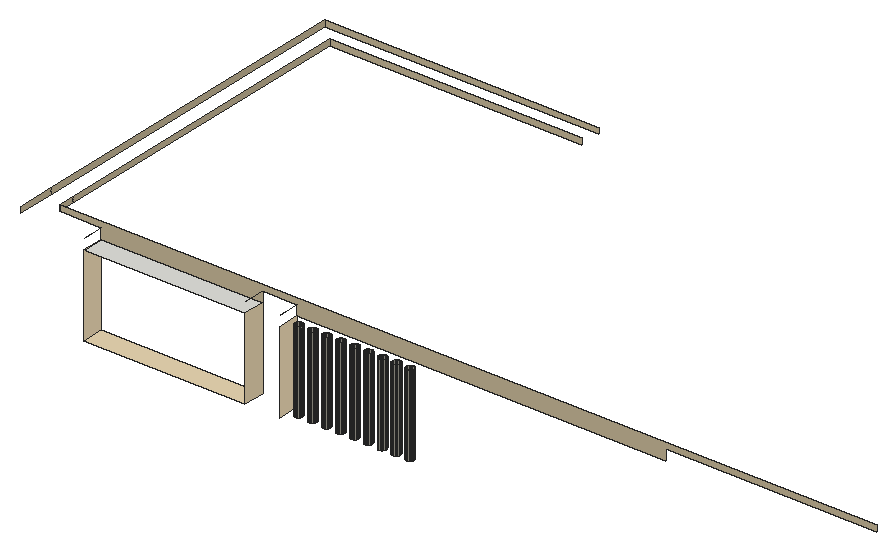
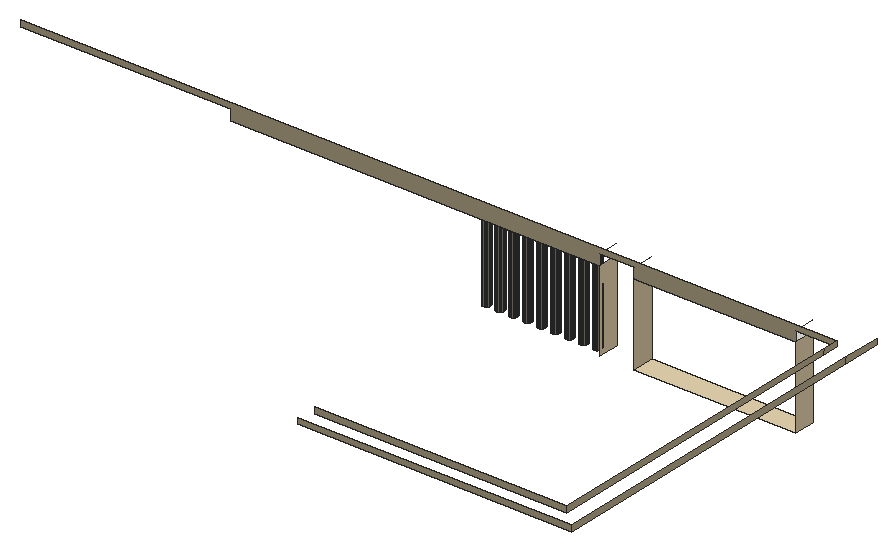
# SketchUp Ruby script. Lengths in inches.
U = 1.inch
M = Sketchup.active_model
def pt(a) = Geom::Point3d.new(a.map { |v| v * U })
def face(e, loops, mat)
  f = e.add_face(loops[0].map { |a| pt(a) })
  loops[1..].each { |l| e.add_face(l.map { |a| pt(a) }).erase! }
  f.material = f.back_material = mat if mat
  f
end
# faces: each face lists its corners as indices into pts; further lists are holes
def faces(e, pts, list, mat = nil) = list.each { |f| face(e, (f[0].is_a?(Array) ? f : [f]).map { |l| l.map { |i| pts[i] } }, mat) }
# xy, xz, yz: faces in a plane at the given z, y or x. An outline is a flat list of corners, or four numbers for a rectangle; further outlines are holes
def ring(l) = l.size == 4 ? [[l[0], l[1]], [l[2], l[1]], [l[2], l[3]], [l[0], l[3]]] : l.each_slice(2).to_a
def flat(e, list, mat, &to3) = list.each { |f| face(e, (f[0].is_a?(Array) ? f : [f]).map { |l| ring(l).map { |u, v| to3.(u, v) } }, mat) }
def xy(e, z, list, mat = nil) = flat(e, list, mat) { |x, y| [x, y, z] }
def xz(e, y, list, mat = nil) = flat(e, list, mat) { |x, z| [x, y, z] }
def yz(e, x, list, mat = nil) = flat(e, list, mat) { |y, z| [x, y, z] }
def lines(e, pts, list) = list.each { |a, b| e.add_line(pt(pts[a]), pt(pts[b])) }
# prism: a flat outline (further loops are holes) pulled along v
def prism(e, loops, v, mat = nil)
  f = face(e, loops, mat); d = Geom::Vector3d.new(v.map { |x| x * U })
  f.pushpull(f.normal.samedirection?(d) ? d.length : -d.length)
end
def box(e, o, s, mat = nil) = prism(e, [[o, [o[0] + s[0], o[1], o[2]], [o[0] + s[0], o[1] + s[1], o[2]], [o[0], o[1] + s[1], o[2]]]], [0, 0, s[2]], mat)
def at(x, y, z, deg = 0) = Geom::Transformation.translation(pt([x, y, z])) * Geom::Transformation.rotation(ORIGIN, Z_AXIS, deg.degrees)
def axes(o, x, y, z) = Geom::Transformation.new([*x, 0, *y, 0, *z, 0, *pt(o).to_a, 1])
def part(name) = M.definitions.add(name)
# library, detail: a bought-in or finely detailed component or shape, given as its bounding box
def library(name, o, s) = part(name).tap { |d| box(d.entities, o, s) }
def detail(e, o, s) = box(e.add_group.entities, o, s)
def put(e, d, t, mat = nil) = e.add_instance(d, t).tap { |i| i.material = mat if mat }
def group(e, t, mat = nil) = e.add_group.tap { |g| g.transformation = t; g.material = mat if mat }.entities
root = M.entities
M.materials.add("[Formica Graystone]").color = [149, 146, 135]
M.materials.add("[Quartz Light Brown]").color = [242, 223, 185]
M.materials.add("[Quartz Light Brown]1").color = [234, 216, 179]
M.materials.add("[Quartz Light Brown]2").color = [199, 184, 152]
xy(root,552.75,[[185.125,21.93,184.41,22.02,183.75,22.3,183.18,22.74,182.74,23.3,182.47,23.97,182.375,24.68,182.47,25.39,182.74,26.05,183.18,26.625,183.75,27.0625,184.41,27.34,185.125,27.43,185.84,27.34,186.5,27.0625,187.07,26.625,187.51,26.05,187.78,25.39,187.875,24.68,187.78,23.97,187.51,23.3,187.07,22.74,186.5,22.3,185.84,22.02],[194.6875,21.93,193.98,22.02,193.3125,22.3,192.74,22.74,192.31,23.3,192.03,23.97,191.9375,24.68,192.03,25.39,192.31,26.05,192.74,26.625,193.3125,27.0625,193.98,27.34,194.6875,27.43,195.4,27.34,196.0625,27.0625,196.63,26.625,197.07,26.05,197.34,25.39,197.4375,24.68,197.34,23.97,197.07,23.3,196.63,22.74,196.0625,22.3,195.4,22.02],[204.25,21.93,203.54,22.02,202.875,22.3,202.31,22.74,201.87,23.3,201.59,23.97,201.5,24.68,201.59,25.39,201.87,26.05,202.31,26.625,202.875,27.0625,203.54,27.34,204.25,27.43,204.96,27.34,205.625,27.0625,206.19,26.625,206.63,26.05,206.91,25.39,207,24.68,206.91,23.97,206.63,23.3,206.19,22.74,205.625,22.3,204.96,22.02],[213.8125,21.93,213.1,22.02,212.4375,22.3,211.87,22.74,211.43,23.3,211.16,23.97,211.0625,24.68,211.16,25.39,211.43,26.05,211.87,26.625,212.4375,27.0625,213.1,27.34,213.8125,27.43,214.52,27.34,215.1875,27.0625,215.76,26.625,216.19,26.05,216.47,25.39,216.5625,24.68,216.47,23.97,216.19,23.3,215.76,22.74,215.1875,22.3,214.52,22.02],[223.375,21.93,222.66,22.02,222,22.3,221.43,22.74,220.99,23.3,220.72,23.97,220.625,24.68,220.72,25.39,220.99,26.05,221.43,26.625,222,27.0625,222.66,27.34,223.375,27.43,224.09,27.34,224.75,27.0625,225.32,26.625,225.76,26.05,226.03,25.39,226.125,24.68,226.03,23.97,225.76,23.3,225.32,22.74,224.75,22.3,224.09,22.02],
  [232.9375,21.93,232.23,22.02,231.5625,22.3,230.99,22.74,230.56,23.3,230.28,23.97,230.1875,24.68,230.28,25.39,230.56,26.05,230.99,26.625,231.5625,27.0625,232.23,27.34,232.9375,27.43,233.65,27.34,234.3125,27.0625,234.88,26.625,235.32,26.05,235.59,25.39,235.6875,24.68,235.59,23.97,235.32,23.3,234.88,22.74,234.3125,22.3,233.65,22.02],[242.5,21.93,241.79,22.02,241.125,22.3,240.56,22.74,240.12,23.3,239.84,23.97,239.75,24.68,239.84,25.39,240.12,26.05,240.56,26.625,241.125,27.0625,241.79,27.34,242.5,27.43,243.21,27.34,243.875,27.0625,244.44,26.625,244.88,26.05,245.16,25.39,245.25,24.68,245.16,23.97,244.88,23.3,244.44,22.74,243.875,22.3,243.21,22.02],[252.0625,21.93,251.35,22.02,250.6875,22.3,250.12,22.74,249.68,23.3,249.41,23.97,249.3125,24.68,249.41,25.39,249.68,26.05,250.12,26.625,250.6875,27.0625,251.35,27.34,252.0625,27.43,252.77,27.34,253.4375,27.0625,254.01,26.625,254.44,26.05,254.72,25.39,254.8125,24.68,254.72,23.97,254.44,23.3,254.01,22.74,253.4375,22.3,252.77,22.02],[261.625,21.93,260.91,22.02,260.25,22.3,259.68,22.74,259.24,23.3,258.97,23.97,258.875,24.68,258.97,25.39,259.24,26.05,259.68,26.625,260.25,27.0625,260.91,27.34,261.625,27.43,262.34,27.34,263,27.0625,263.57,26.625,264.01,26.05,264.28,25.39,264.375,24.68,264.28,23.97,264.01,23.3,263.57,22.74,263,22.3,262.34,22.02]])
xy(root,552.75,[[43.82,16.1875,154.82,31.11]],"[Quartz Light Brown]1")
xy(root,608.75,[[43.82,16.1875,154.82,31.11]])
xz(root,31.11,[[43.82,608.75,43.82,616,14.92,616,14.92,619.9375,577.38,619.9375,577.38,616,432.54,616,432.54,608.75,178.73,608.75,178.73,616,154.82,616,154.82,608.75]],"[Quartz Light Brown]2")
xz(root,263.56,[[14.92,616,188.57,619.9375]],"[Quartz Light Brown]2")
xz(root,278.48,[[0,616,188.57,619.9375]],"[Quartz Light Brown]2")
yz(root,0,[[16.1875,616,42.53,619.9375],[42.53,616,278.48,619.9375]],"[Quartz Light Brown]2")
yz(root,14.92,[[31.11,616,42.53,619.9375],[42.53,616,263.56,619.9375]],"[Quartz Light Brown]2")
yz(root,43.82,[[16.1875,552.75,31.11,608.75]],"[Quartz Light Brown]")
yz(root,154.82,[[16.1875,552.75,31.11,608.75]],"[Quartz Light Brown]1")
yz(root,178.73,[[16.1875,552.75,31.11,608.75]],"[Quartz Light Brown]")
p = [[184.41,22.02,552.75],[185.125,21.93,552.75],[185.125,21.93,608.75],[184.41,22.02,608.75],[185.84,22.02,552.75],[185.84,22.02,608.75],
  [193.98,22.02,552.75],[194.6875,21.93,552.75],[194.6875,21.93,608.75],[193.98,22.02,608.75],[195.4,22.02,552.75],[195.4,22.02,608.75],
  [203.54,22.02,552.75],[204.25,21.93,552.75],[204.25,21.93,608.75],[203.54,22.02,608.75],[204.96,22.02,552.75],[204.96,22.02,608.75],
  [213.1,22.02,552.75],[213.8125,21.93,552.75],[213.8125,21.93,608.75],[213.1,22.02,608.75],[214.52,22.02,552.75],[214.52,22.02,608.75],
  [222.66,22.02,552.75],[223.375,21.93,552.75],[223.375,21.93,608.75],[222.66,22.02,608.75],[224.09,22.02,552.75],[224.09,22.02,608.75],
  [232.23,22.02,552.75],[232.9375,21.93,552.75],[232.9375,21.93,608.75],[232.23,22.02,608.75],[233.65,22.02,552.75],[233.65,22.02,608.75],
  [241.79,22.02,552.75],[242.5,21.93,552.75],[242.5,21.93,608.75],[241.79,22.02,608.75],[243.21,22.02,552.75],[243.21,22.02,608.75],
  [251.35,22.02,552.75],[252.0625,21.93,552.75],[252.0625,21.93,608.75],[251.35,22.02,608.75],[252.77,22.02,552.75],[252.77,22.02,608.75],
  [260.91,22.02,552.75],[261.625,21.93,552.75],[261.625,21.93,608.75],[260.91,22.02,608.75],[262.34,22.02,552.75],[262.34,22.02,608.75],
  [183.75,22.3,552.75],[183.75,22.3,608.75],[186.5,22.3,552.75],[186.5,22.3,608.75],[193.3125,22.3,552.75],[193.3125,22.3,608.75],
  [196.0625,22.3,552.75],[196.0625,22.3,608.75],[202.875,22.3,552.75],[202.875,22.3,608.75],[205.625,22.3,552.75],[205.625,22.3,608.75],
  [212.4375,22.3,552.75],[212.4375,22.3,608.75],[215.1875,22.3,552.75],[215.1875,22.3,608.75],[222,22.3,552.75],[222,22.3,608.75],
  [224.75,22.3,552.75],[224.75,22.3,608.75],[231.5625,22.3,552.75],[231.5625,22.3,608.75],[234.3125,22.3,552.75],[234.3125,22.3,608.75],
  [241.125,22.3,552.75],[241.125,22.3,608.75],[243.875,22.3,552.75],[243.875,22.3,608.75],[250.6875,22.3,552.75],[250.6875,22.3,608.75],
  [253.4375,22.3,552.75],[253.4375,22.3,608.75],[260.25,22.3,552.75],[260.25,22.3,608.75],[263,22.3,552.75],[263,22.3,608.75],
  [183.18,22.74,552.75],[183.18,22.74,608.75],[187.07,22.74,552.75],[187.07,22.74,608.75],[192.74,22.74,552.75],[192.74,22.74,608.75],
  [196.63,22.74,552.75],[196.63,22.74,608.75],[202.31,22.74,552.75],[202.31,22.74,608.75],[206.19,22.74,552.75],[206.19,22.74,608.75],
  [211.87,22.74,552.75],[211.87,22.74,608.75],[215.76,22.74,552.75],[215.76,22.74,608.75],[221.43,22.74,552.75],[221.43,22.74,608.75],
  [225.32,22.74,552.75],[225.32,22.74,608.75],[230.99,22.74,552.75],[230.99,22.74,608.75],[234.88,22.74,552.75],[234.88,22.74,608.75],
  [240.56,22.74,552.75],[240.56,22.74,608.75],[244.44,22.74,552.75],[244.44,22.74,608.75],[250.12,22.74,552.75],[250.12,22.74,608.75],
  [254.01,22.74,552.75],[254.01,22.74,608.75],[259.68,22.74,552.75],[259.68,22.74,608.75],[263.57,22.74,552.75],[263.57,22.74,608.75],
  [182.74,23.3,552.75],[182.74,23.3,608.75],[187.51,23.3,552.75],[187.51,23.3,608.75],[192.31,23.3,552.75],[192.31,23.3,608.75],
  [197.07,23.3,552.75],[197.07,23.3,608.75],[201.87,23.3,552.75],[201.87,23.3,608.75],[206.63,23.3,552.75],[206.63,23.3,608.75],
  [211.43,23.3,552.75],[211.43,23.3,608.75],[216.19,23.3,552.75],[216.19,23.3,608.75],[220.99,23.3,552.75],[220.99,23.3,608.75],
  [225.76,23.3,552.75],[225.76,23.3,608.75],[230.56,23.3,552.75],[230.56,23.3,608.75],[235.32,23.3,552.75],[235.32,23.3,608.75],
  [240.12,23.3,552.75],[240.12,23.3,608.75],[244.88,23.3,552.75],[244.88,23.3,608.75],[249.68,23.3,552.75],[249.68,23.3,608.75],
  [254.44,23.3,552.75],[254.44,23.3,608.75],[259.24,23.3,552.75],[259.24,23.3,608.75],[264.01,23.3,552.75],[264.01,23.3,608.75],
  [182.47,23.97,552.75],[182.47,23.97,608.75],[187.78,23.97,552.75],[187.78,23.97,608.75],[192.03,23.97,552.75],[192.03,23.97,608.75],
  [197.34,23.97,552.75],[197.34,23.97,608.75],[201.59,23.97,552.75],[201.59,23.97,608.75],[206.91,23.97,552.75],[206.91,23.97,608.75],
  [211.16,23.97,552.75],[211.16,23.97,608.75],[216.47,23.97,552.75],[216.47,23.97,608.75],[220.72,23.97,552.75],[220.72,23.97,608.75],
  [226.03,23.97,552.75],[226.03,23.97,608.75],[230.28,23.97,552.75],[230.28,23.97,608.75],[235.59,23.97,552.75],[235.59,23.97,608.75],
  [239.84,23.97,552.75],[239.84,23.97,608.75],[245.16,23.97,552.75],[245.16,23.97,608.75],[249.41,23.97,552.75],[249.41,23.97,608.75],
  [254.72,23.97,552.75],[254.72,23.97,608.75],[258.97,23.97,552.75],[258.97,23.97,608.75],[264.28,23.97,552.75],[264.28,23.97,608.75],
  [182.375,24.68,552.75],[182.375,24.68,608.75],[187.875,24.68,552.75],[187.875,24.68,608.75],[191.9375,24.68,552.75],[191.9375,24.68,608.75],
  [197.4375,24.68,552.75],[197.4375,24.68,608.75],[201.5,24.68,552.75],[201.5,24.68,608.75],[207,24.68,552.75],[207,24.68,608.75],
  [211.0625,24.68,552.75],[211.0625,24.68,608.75],[216.5625,24.68,552.75],[216.5625,24.68,608.75],[220.625,24.68,552.75],[220.625,24.68,608.75],
  [226.125,24.68,552.75],[226.125,24.68,608.75],[230.1875,24.68,552.75],[230.1875,24.68,608.75],[235.6875,24.68,552.75],[235.6875,24.68,608.75],
  [239.75,24.68,552.75],[239.75,24.68,608.75],[245.25,24.68,552.75],[245.25,24.68,608.75],[249.3125,24.68,552.75],[249.3125,24.68,608.75],
  [254.8125,24.68,552.75],[254.8125,24.68,608.75],[258.875,24.68,552.75],[258.875,24.68,608.75],[264.375,24.68,552.75],[264.375,24.68,608.75],
  [182.47,25.39,552.75],[182.47,25.39,608.75],[187.78,25.39,552.75],[187.78,25.39,608.75],[192.03,25.39,552.75],[192.03,25.39,608.75],
  [197.34,25.39,552.75],[197.34,25.39,608.75],[201.59,25.39,552.75],[201.59,25.39,608.75],[206.91,25.39,552.75],[206.91,25.39,608.75],
  [211.16,25.39,552.75],[211.16,25.39,608.75],[216.47,25.39,552.75],[216.47,25.39,608.75],[220.72,25.39,552.75],[220.72,25.39,608.75],
  [226.03,25.39,552.75],[226.03,25.39,608.75],[230.28,25.39,552.75],[230.28,25.39,608.75],[235.59,25.39,552.75],[235.59,25.39,608.75],
  [239.84,25.39,552.75],[239.84,25.39,608.75],[245.16,25.39,552.75],[245.16,25.39,608.75],[249.41,25.39,552.75],[249.41,25.39,608.75],
  [254.72,25.39,552.75],[254.72,25.39,608.75],[258.97,25.39,552.75],[258.97,25.39,608.75],[264.28,25.39,552.75],[264.28,25.39,608.75],
  [182.74,26.05,552.75],[182.74,26.05,608.75],[187.51,26.05,552.75],[187.51,26.05,608.75],[192.31,26.05,552.75],[192.31,26.05,608.75],
  [197.07,26.05,552.75],[197.07,26.05,608.75],[201.87,26.05,552.75],[201.87,26.05,608.75],[206.63,26.05,552.75],[206.63,26.05,608.75],
  [211.43,26.05,552.75],[211.43,26.05,608.75],[216.19,26.05,552.75],[216.19,26.05,608.75],[220.99,26.05,552.75],[220.99,26.05,608.75],
  [225.76,26.05,552.75],[225.76,26.05,608.75],[230.56,26.05,552.75],[230.56,26.05,608.75],[235.32,26.05,552.75],[235.32,26.05,608.75],
  [240.12,26.05,552.75],[240.12,26.05,608.75],[244.88,26.05,552.75],[244.88,26.05,608.75],[249.68,26.05,552.75],[249.68,26.05,608.75],
  [254.44,26.05,552.75],[254.44,26.05,608.75],[259.24,26.05,552.75],[259.24,26.05,608.75],[264.01,26.05,552.75],[264.01,26.05,608.75],
  [183.18,26.625,552.75],[183.18,26.625,608.75],[187.07,26.625,552.75],[187.07,26.625,608.75],[192.74,26.625,552.75],[192.74,26.625,608.75],
  [196.63,26.625,552.75],[196.63,26.625,608.75],[202.31,26.625,552.75],[202.31,26.625,608.75],[206.19,26.625,552.75],[206.19,26.625,608.75],
  [211.87,26.625,552.75],[211.87,26.625,608.75],[215.76,26.625,552.75],[215.76,26.625,608.75],[221.43,26.625,552.75],[221.43,26.625,608.75],
  [225.32,26.625,552.75],[225.32,26.625,608.75],[230.99,26.625,552.75],[230.99,26.625,608.75],[234.88,26.625,552.75],[234.88,26.625,608.75],
  [240.56,26.625,552.75],[240.56,26.625,608.75],[244.44,26.625,552.75],[244.44,26.625,608.75],[250.12,26.625,552.75],[250.12,26.625,608.75],
  [254.01,26.625,552.75],[254.01,26.625,608.75],[259.68,26.625,552.75],[259.68,26.625,608.75],[263.57,26.625,552.75],[263.57,26.625,608.75],
  [183.75,27.0625,552.75],[183.75,27.0625,608.75],[186.5,27.0625,552.75],[186.5,27.0625,608.75],[193.3125,27.0625,552.75],[193.3125,27.0625,608.75],
  [196.0625,27.0625,552.75],[196.0625,27.0625,608.75],[202.875,27.0625,552.75],[202.875,27.0625,608.75],[205.625,27.0625,552.75],[205.625,27.0625,608.75],
  [212.4375,27.0625,552.75],[212.4375,27.0625,608.75],[215.1875,27.0625,552.75],[215.1875,27.0625,608.75],[222,27.0625,552.75],[222,27.0625,608.75],
  [224.75,27.0625,552.75],[224.75,27.0625,608.75],[231.5625,27.0625,552.75],[231.5625,27.0625,608.75],[234.3125,27.0625,552.75],[234.3125,27.0625,608.75],
  [241.125,27.0625,552.75],[241.125,27.0625,608.75],[243.875,27.0625,552.75],[243.875,27.0625,608.75],[250.6875,27.0625,552.75],[250.6875,27.0625,608.75],
  [253.4375,27.0625,552.75],[253.4375,27.0625,608.75],[260.25,27.0625,552.75],[260.25,27.0625,608.75],[263,27.0625,552.75],[263,27.0625,608.75],
  [184.41,27.34,552.75],[184.41,27.34,608.75],[185.84,27.34,552.75],[185.84,27.34,608.75],[193.98,27.34,552.75],[193.98,27.34,608.75],
  [195.4,27.34,552.75],[195.4,27.34,608.75],[203.54,27.34,552.75],[203.54,27.34,608.75],[204.96,27.34,552.75],[204.96,27.34,608.75],
  [213.1,27.34,552.75],[213.1,27.34,608.75],[214.52,27.34,552.75],[214.52,27.34,608.75],[222.66,27.34,552.75],[222.66,27.34,608.75],
  [224.09,27.34,552.75],[224.09,27.34,608.75],[232.23,27.34,552.75],[232.23,27.34,608.75],[233.65,27.34,552.75],[233.65,27.34,608.75],
  [241.79,27.34,552.75],[241.79,27.34,608.75],[243.21,27.34,552.75],[243.21,27.34,608.75],[251.35,27.34,552.75],[251.35,27.34,608.75],
  [252.77,27.34,552.75],[252.77,27.34,608.75],[260.91,27.34,552.75],[260.91,27.34,608.75],[262.34,27.34,552.75],[262.34,27.34,608.75],
  [185.125,27.43,552.75],[185.125,27.43,608.75],[194.6875,27.43,552.75],[194.6875,27.43,608.75],[204.25,27.43,552.75],[204.25,27.43,608.75],
  [213.8125,27.43,552.75],[213.8125,27.43,608.75],[223.375,27.43,552.75],[223.375,27.43,608.75],[232.9375,27.43,552.75],[232.9375,27.43,608.75],
  [242.5,27.43,552.75],[242.5,27.43,608.75],[252.0625,27.43,552.75],[252.0625,27.43,608.75],[261.625,27.43,552.75],[261.625,27.43,608.75],
  [43.82,16.1875,616],[43.82,31.11,616],[154.82,16.1875,616],[154.82,31.11,616],[178.73,31.11,616],[178.73,16.1875,616]]
faces(root,p,[[0,1,2,3],[1,4,5,2],[6,7,8,9],[7,10,11,8],[12,13,14,15],[13,16,17,14],[18,19,20,21],[19,22,23,20],
  [24,25,26,27],[25,28,29,26],[30,31,32,33],[31,34,35,32],[36,37,38,39],[37,40,41,38],[42,43,44,45],[43,46,47,44],
  [48,49,50,51],[49,52,53,50],[54,0,3,55],[4,56,57,5],[58,6,9,59],[10,60,61,11],[62,12,15,63],[16,64,65,17],
  [66,18,21,67],[22,68,69,23],[70,24,27,71],[28,72,73,29],[74,30,33,75],[34,76,77,35],[78,36,39,79],[40,80,81,41],
  [82,42,45,83],[46,84,85,47],[86,48,51,87],[52,88,89,53],[90,54,55,91],[56,92,93,57],[94,58,59,95],[60,96,97,61],
  [98,62,63,99],[64,100,101,65],[102,66,67,103],[68,104,105,69],[106,70,71,107],[72,108,109,73],[110,74,75,111],[76,112,113,77],
  [114,78,79,115],[80,116,117,81],[118,82,83,119],[84,120,121,85],[122,86,87,123],[88,124,125,89],[126,90,91,127],[92,128,129,93],
  [130,94,95,131],[96,132,133,97],[134,98,99,135],[100,136,137,101],[138,102,103,139],[104,140,141,105],[142,106,107,143],[108,144,145,109],
  [146,110,111,147],[112,148,149,113],[150,114,115,151],[116,152,153,117],[154,118,119,155],[120,156,157,121],[158,122,123,159],[124,160,161,125],
  [162,126,127,163],[128,164,165,129],[166,130,131,167],[132,168,169,133],[170,134,135,171],[136,172,173,137],[174,138,139,175],[140,176,177,141],
  [178,142,143,179],[144,180,181,145],[182,146,147,183],[148,184,185,149],[186,150,151,187],[152,188,189,153],[190,154,155,191],[156,192,193,157],
  [194,158,159,195],[160,196,197,161],[198,162,163,199],[164,200,201,165],[202,166,167,203],[168,204,205,169],[206,170,171,207],[172,208,209,173],
  [210,174,175,211],[176,212,213,177],[214,178,179,215],[180,216,217,181],[218,182,183,219],[184,220,221,185],[222,186,187,223],[188,224,225,189],
  [226,190,191,227],[192,228,229,193],[230,194,195,231],[196,232,233,197],[234,198,199,235],[200,236,237,201],[238,202,203,239],[204,240,241,205],
  [242,206,207,243],[208,244,245,209],[246,210,211,247],[212,248,249,213],[250,214,215,251],[216,252,253,217],[254,218,219,255],[220,256,257,221],
  [258,222,223,259],[224,260,261,225],[262,226,227,263],[228,264,265,229],[266,230,231,267],[232,268,269,233],[270,234,235,271],[236,272,273,237],
  [274,238,239,275],[240,276,277,241],[278,242,243,279],[244,280,281,245],[282,246,247,283],[248,284,285,249],[286,250,251,287],[252,288,289,253],
  [290,254,255,291],[256,292,293,257],[294,258,259,295],[260,296,297,261],[298,262,263,299],[264,300,301,265],[302,266,267,303],[268,304,305,269],
  [306,270,271,307],[272,308,309,273],[310,274,275,311],[276,312,313,277],[314,278,279,315],[280,316,317,281],[318,282,283,319],[284,320,321,285],
  [322,286,287,323],[288,324,325,289],[326,290,291,327],[292,328,329,293],[330,294,295,331],[296,332,333,297],[334,298,299,335],[300,336,337,301],
  [338,302,303,339],[304,340,341,305],[342,306,307,343],[308,344,345,309],[346,310,311,347],[312,348,349,313],[350,314,315,351],[316,352,353,317],
  [354,318,319,355],[320,356,357,321],[358,322,323,359],[324,360,361,325],[362,326,327,363],[328,364,365,329],[366,330,331,367],[332,368,369,333],
  [370,334,335,371],[336,372,373,337],[374,338,339,375],[340,376,377,341],[378,342,343,379],[344,380,381,345],[382,346,347,383],[348,384,385,349],
  [386,350,351,387],[352,388,389,353],[390,354,355,391],[356,392,393,357],[394,358,359,395],[360,396,397,361],[398,362,363,399],[364,400,401,365],
  [402,366,367,403],[368,404,405,369],[406,370,371,407],[372,408,409,373],[410,374,375,411],[376,412,413,377],[414,378,379,415],[380,414,415,381],
  [416,382,383,417],[384,416,417,385],[418,386,387,419],[388,418,419,389],[420,390,391,421],[392,420,421,393],[422,394,395,423],[396,422,423,397],
  [424,398,399,425],[400,424,425,401],[426,402,403,427],[404,426,427,405],[428,406,407,429],[408,428,429,409],[430,410,411,431],[412,430,431,413]],"[Formica Graystone]")
lines(root,p,[[432,433],[434,435],[436,437]])
